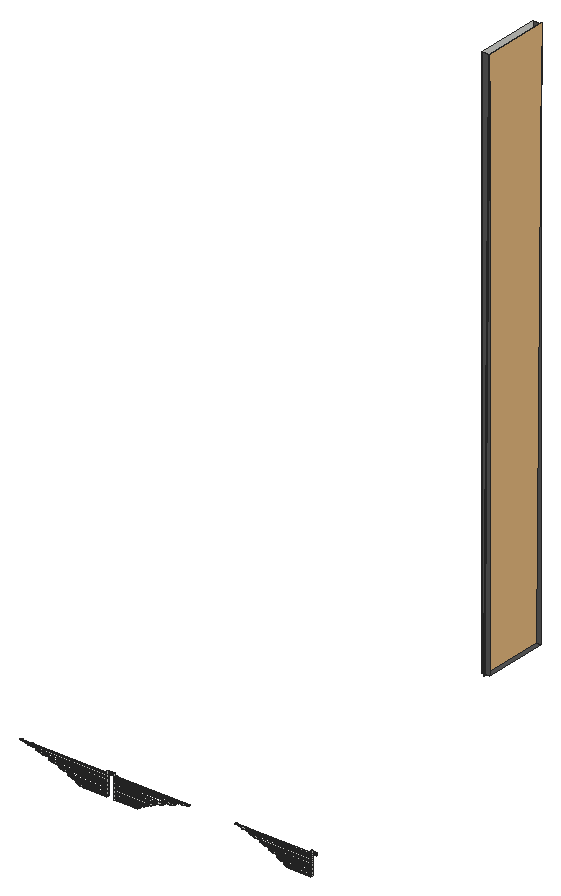
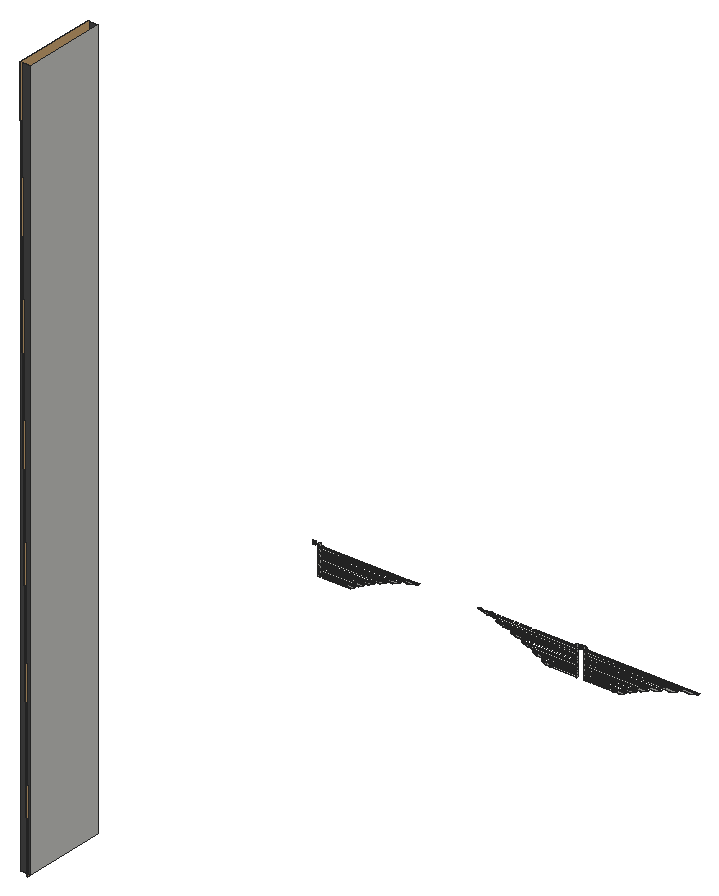
# SketchUp Ruby script. Lengths in inches.
U = 1.inch
M = Sketchup.active_model
def pt(a) = Geom::Point3d.new(a.map { |v| v * U })
def face(e, loops, mat)
  f = e.add_face(loops[0].map { |a| pt(a) })
  loops[1..].each { |l| e.add_face(l.map { |a| pt(a) }).erase! }
  f.material = f.back_material = mat if mat
  f
end
# faces: each face lists its corners as indices into pts; further lists are holes
def faces(e, pts, list, mat = nil) = list.each { |f| face(e, (f[0].is_a?(Array) ? f : [f]).map { |l| l.map { |i| pts[i] } }, mat) }
# xy, xz, yz: faces in a plane at the given z, y or x. An outline is a flat list of corners, or four numbers for a rectangle; further outlines are holes
def ring(l) = l.size == 4 ? [[l[0], l[1]], [l[2], l[1]], [l[2], l[3]], [l[0], l[3]]] : l.each_slice(2).to_a
def flat(e, list, mat, &to3) = list.each { |f| face(e, (f[0].is_a?(Array) ? f : [f]).map { |l| ring(l).map { |u, v| to3.(u, v) } }, mat) }
def xy(e, z, list, mat = nil) = flat(e, list, mat) { |x, y| [x, y, z] }
def xz(e, y, list, mat = nil) = flat(e, list, mat) { |x, z| [x, y, z] }
def yz(e, x, list, mat = nil) = flat(e, list, mat) { |y, z| [x, y, z] }
def lines(e, pts, list) = list.each { |a, b| e.add_line(pt(pts[a]), pt(pts[b])) }
# prism: a flat outline (further loops are holes) pulled along v
def prism(e, loops, v, mat = nil)
  f = face(e, loops, mat); d = Geom::Vector3d.new(v.map { |x| x * U })
  f.pushpull(f.normal.samedirection?(d) ? d.length : -d.length)
end
def box(e, o, s, mat = nil) = prism(e, [[o, [o[0] + s[0], o[1], o[2]], [o[0] + s[0], o[1] + s[1], o[2]], [o[0], o[1] + s[1], o[2]]]], [0, 0, s[2]], mat)
def at(x, y, z, deg = 0) = Geom::Transformation.translation(pt([x, y, z])) * Geom::Transformation.rotation(ORIGIN, Z_AXIS, deg.degrees)
def axes(o, x, y, z) = Geom::Transformation.new([*x, 0, *y, 0, *z, 0, *pt(o).to_a, 1])
def part(name) = M.definitions.add(name)
# library, detail: a bought-in or finely detailed component or shape, given as its bounding box
def library(name, o, s) = part(name).tap { |d| box(d.entities, o, s) }
def detail(e, o, s) = box(e.add_group.entities, o, s)
def put(e, d, t, mat = nil) = e.add_instance(d, t).tap { |i| i.material = mat if mat }
def group(e, t, mat = nil) = e.add_group.tap { |g| g.transformation = t; g.material = mat if mat }.entities
root = M.entities
M.materials.add("[Color M06]").color = [86, 86, 86]
c1 = library("Big Leaf.dwg\#1",[0,0,0],[43.17,84,0.75])
xy(root,27.6875,[[968.64,12.93,975.85,13.56],[975.85,12.93,1012.48,13.56],[1024.39,12.93,1056.27,13.56],[1056.27,12.93,1062.53,13.56],[1307.3125,12.93,1313.58,13.56],
  [1313.58,12.93,1345.46,13.56],[968.64,13.81,975.85,14.31],[975.85,13.81,1012.48,14.31],[1024.39,13.81,1056.27,14.31],[1056.27,13.81,1062.53,14.31],
  [1307.3125,13.81,1313.58,14.31],[1313.58,13.81,1345.46,14.31]])
xy(root,28.18,[[967.85,12.93,975.85,14.31],[975.85,12.93,1013.27,14.31],[1023.71,12.93,1056.27,14.31],[1056.27,12.93,1063.22,14.31],[1306.63,12.93,1313.58,14.31],
  [1313.58,12.93,1346.14,14.31]])
xy(root,30.61,[[963.14,12.93,971.13,14.31],[971.13,12.93,1013.27,14.31],[1023.71,12.93,1060.36,14.31],[1060.36,12.93,1067.32,14.31],[1302.53,12.93,1309.48,14.31],
  [1309.48,12.93,1346.14,14.31]])
xy(root,31.1,[[962.35,12.93,971.13,13.56],[971.13,12.93,1012.48,13.56],[1024.39,12.93,1060.36,13.56],[1060.36,12.93,1068,13.56],[1301.84,12.93,1309.48,13.56],
  [1309.48,12.93,1345.46,13.56],[962.35,13.81,971.13,14.31],[971.13,13.81,1012.48,14.31],[1024.39,13.81,1060.36,14.31],[1060.36,13.81,1068,14.31],
  [1301.84,13.81,1309.48,14.31],[1309.48,13.81,1345.46,14.31]])
xy(root,31.9,[[1189.6875,557.39,1202.5625,662.57]],"[Color M06]")
xy(root,33.81,[[956.23,12.93,963.95,13.56],[963.95,12.93,1012.48,13.56],[1024.39,12.93,1066.61,13.56],[1066.61,12.93,1073.33,13.56],[1296.52,12.93,1303.24,13.56],
  [1303.24,12.93,1345.46,13.56],[956.23,13.81,963.95,14.31],[963.95,13.81,1012.48,14.31],[1024.39,13.81,1066.61,14.31],[1066.61,13.81,1073.33,14.31],
  [1296.52,13.81,1303.24,14.31],[1303.24,13.81,1345.46,14.31]])
xy(root,34.3,[[955.44,12.93,963.95,14.31],[963.95,12.93,1013.27,14.31],[1023.71,12.93,1066.61,14.31],[1066.61,12.93,1074.02,14.31],[1295.83,12.93,1303.24,14.31],
  [1303.24,12.93,1346.14,14.31]])
xy(root,36.73,[[950.1,12.93,958.75,14.31],[958.75,12.93,1013.27,14.31],[1023.71,12.93,1071.14,14.31],[1071.14,12.93,1078.67,14.31],[1291.18,12.93,1298.7,14.31],
  [1298.7,12.93,1346.14,14.31]])
xy(root,37.22,[[949.3125,12.93,958.75,13.56],[958.75,12.93,1012.48,13.56],[1024.39,12.93,1071.14,13.56],[1071.14,12.93,1079.35,13.56],[1290.5,12.93,1298.7,13.56],
  [1298.7,12.93,1345.46,13.56],[949.3125,13.81,958.75,14.31],[958.75,13.81,1012.48,14.31],[1024.39,13.81,1071.14,14.31],[1071.14,13.81,1079.35,14.31],
  [1290.5,13.81,1298.7,14.31],[1298.7,13.81,1345.46,14.31]])
xy(root,39.93,[[942.21,12.93,950.6,13.56],[950.6,12.93,1012.48,13.56],[1024.39,12.93,1078.23,13.56],[1078.23,12.93,1085.53,13.56],[1284.32,12.93,1291.62,13.56],
  [1291.62,12.93,1345.46,13.56],[942.21,13.81,950.6,14.31],[950.6,13.81,1012.48,14.31],[1024.39,13.81,1078.23,14.31],[1078.23,13.81,1085.53,14.31],
  [1284.32,13.81,1291.62,14.31],[1291.62,13.81,1345.46,14.31]])
xy(root,40.42,[[941.43,12.93,950.6,14.31],[950.6,12.93,1013.27,14.31],[1023.71,12.93,1078.23,14.31],[1078.23,12.93,1086.21,14.31],[1283.64,12.93,1291.62,14.31],
  [1291.62,12.93,1346.14,14.31]])
xy(root,42.85,[[935.33,12.93,944.79,14.31],[944.79,12.93,1013.27,14.31],[1023.71,12.93,1083.28,14.31],[1083.28,12.93,1091.51,14.31],[1278.34,12.93,1286.57,14.31],
  [1286.57,12.93,1346.14,14.31]])
xy(root,43.34,[[934.55,12.93,944.79,13.56],[944.79,12.93,1012.48,13.56],[1024.39,12.93,1083.28,13.56],[1083.28,12.93,1092.19,13.56],[1277.65,12.93,1286.57,13.56],
  [1286.57,12.93,1345.46,13.56],[934.55,13.81,944.79,14.31],[944.79,13.81,1012.48,14.31],[1024.39,13.81,1083.28,14.31],[1083.28,13.81,1092.19,14.31],
  [1277.65,13.81,1286.57,14.31],[1286.57,13.81,1345.46,14.31]])
xy(root,46.05,[[926.1,12.93,935.51,13.56],[935.51,12.93,1012.48,13.56],[1024.39,12.93,1091.36,13.56],[1091.36,12.93,1099.55,13.56],[1270.3,12.93,1278.49,13.56],
  [1278.49,12.93,1345.46,13.56],[926.1,13.81,935.51,14.31],[935.51,13.81,1012.48,14.31],[1024.39,13.81,1091.36,14.31],[1091.36,13.81,1099.55,14.31],
  [1270.3,13.81,1278.49,14.31],[1278.49,13.81,1345.46,14.31]])
xy(root,46.54,[[925.31,12.93,935.51,14.31],[935.51,12.93,1013.27,14.31],[1023.71,12.93,1091.36,14.31],[1091.36,12.93,1100.23,14.31],[1269.61,12.93,1278.49,14.31],
  [1278.49,12.93,1346.14,14.31]])
xy(root,48.97,[[918.3125,12.93,928.79,14.31],[928.79,12.93,1013.27,14.31],[1023.71,12.93,1097.2,14.31],[1097.2,12.93,1106.32,14.31],[1263.53,12.93,1272.65,14.31],
  [1272.65,12.93,1346.14,14.31]])
xy(root,49.46,[[917.52,12.93,928.79,13.56],[928.79,12.93,1012.48,13.56],[1024.39,12.93,1097.2,13.56],[1097.2,12.93,1107,13.56],[1262.84,12.93,1272.65,13.56],
  [1272.65,12.93,1345.46,13.56],[917.52,13.81,928.79,14.31],[928.79,13.81,1012.48,14.31],[1024.39,13.81,1097.2,14.31],[1097.2,13.81,1107,14.31],
  [1262.84,13.81,1272.65,14.31],[1272.65,13.81,1345.46,14.31]])
xy(root,52.17,[[907.12,12.93,918.13,13.56],[918.13,12.93,1012.48,13.56],[1024.39,12.93,1106.48,13.56],[1106.48,12.93,1116.06,13.56],[1253.79,12.93,1263.37,13.56],
  [1263.37,12.93,1345.46,13.56],[907.12,13.81,918.13,14.31],[918.13,13.81,1012.48,14.31],[1024.39,13.81,1106.48,14.31],[1106.48,13.81,1116.06,14.31],
  [1253.79,13.81,1263.37,14.31],[1263.37,13.81,1345.46,14.31]])
xy(root,52.67,[[906.33,12.93,918.13,14.31],[918.13,12.93,1013.27,14.31],[1023.71,12.93,1106.48,14.31],[1106.48,12.93,1116.74,14.31],[1253.1,12.93,1263.37,14.31],
  [1263.37,12.93,1346.14,14.31]])
xy(root,55.09,[[897.86,12.93,910,14.31],[910,12.93,1013.27,14.31],[1023.71,12.93,1113.55,14.31],[1113.55,12.93,1124.11,14.31],[1245.73,12.93,1256.3,14.31],
  [1256.3,12.93,1346.14,14.31]])
xy(root,55.59,[[897.07,12.93,910,13.56],[910,12.93,1012.48,13.56],[1024.39,12.93,1113.55,13.56],[1113.55,12.93,1124.8,13.56],[1245.05,12.93,1256.3,13.56],
  [1256.3,12.93,1345.46,13.56],[897.07,13.81,910,14.31],[910,13.81,1012.48,14.31],[1024.39,13.81,1113.55,14.31],[1113.55,13.81,1124.8,14.31],
  [1245.05,13.81,1256.3,14.31],[1256.3,13.81,1345.46,14.31]])
xy(root,58.29,[[884.76,12.93,896.8,13.56],[896.8,12.93,1012.48,13.56],[1024.39,12.93,1125.03,13.56],[1125.03,12.93,1135.51,13.56],[1234.34,12.93,1244.82,13.56],
  [1244.82,12.93,1345.46,13.56],[884.76,13.81,896.8,14.31],[896.8,13.81,1012.48,14.31],[1024.39,13.81,1125.03,14.31],[1125.03,13.81,1135.51,14.31],
  [1234.34,13.81,1244.82,14.31],[1244.82,13.81,1345.46,14.31]])
xy(root,58.79,[[896.8,12.93,1013.27,14.31],[1023.71,12.93,1125.03,14.31],[1244.82,12.93,1346.14,14.31]])
xy(root,61.21,[[871.53,12.93,887.21,14.31],[887.21,12.93,1013.27,14.31],[1023.71,12.93,1133.375,14.31],[1133.375,12.93,1147.02,14.31],[1222.82,12.93,1236.47,14.31],
  [1236.47,12.93,1346.14,14.31]])
xy(root,61.46,[[1014.6875,13.24,1018.58,14.43],[1019.16,13.24,1023.63,14.43],[1351.27,13.24,1355.16,14.43]])
xy(root,61.71,[[870.74,12.93,887.21,13.56],[887.21,12.93,1012.48,13.56],[1024.39,12.93,1133.375,13.56],[1133.375,12.93,1147.71,13.56],[1222.14,12.93,1236.47,13.56],
  [1236.47,12.93,1345.46,13.56],[870.74,13.81,887.21,14.31],[887.21,13.81,1012.48,14.31],[1024.39,13.81,1133.375,14.31],[1133.375,13.81,1147.71,14.31],
  [1222.14,13.81,1236.47,14.31],[1236.47,13.81,1345.46,14.31]])
xy(root,62.75,[[1014.6875,13.24,1018.58,14.43],[1019.16,13.24,1023.63,14.43],[1351.27,13.24,1355.16,14.43]])
xy(root,63.67,[[1014.6875,13.24,1018.58,14.43],[1019.16,13.24,1023.63,14.43],[1351.27,13.24,1355.16,14.43]])
xz(root,12.93,[[967.85,28.18,963.14,30.61,971.13,30.61,975.85,28.18],[1056.27,28.18,1063.22,28.18,1067.32,30.61,1060.36,30.61],[1306.63,28.18,1302.53,30.61,1309.48,30.61,1313.58,28.18],[955.44,34.3,950.1,36.73,958.75,36.73,962.94,34.82,963.95,34.3],[1066.61,34.3,1074.02,34.3,1078.67,36.73,1071.14,36.73,1067.49,34.82],
  [1295.83,34.3,1291.18,36.73,1298.7,36.73,1302.36,34.82,1303.24,34.3],[941.43,40.42,935.33,42.85,944.79,42.85,948.59,41.34,950.6,40.42],[1078.23,40.42,1086.21,40.42,1091.51,42.85,1083.28,42.85,1079.97,41.34],[1283.64,40.42,1278.34,42.85,1286.57,42.85,1289.87,41.34,1291.62,40.42],[925.31,46.54,918.3125,48.97,928.79,48.97,933.64,47.29,935.51,46.54],
  [1091.36,46.54,1100.23,46.54,1106.32,48.97,1097.2,48.97,1092.98,47.29],[1269.61,46.54,1263.53,48.97,1272.65,48.97,1276.86,47.29,1278.49,46.54],[906.33,52.67,900.11,54.52,897.86,55.09,910,55.09,918.13,52.67],[1106.48,52.67,1116.74,52.67,1122.15,54.52,1124.11,55.09,1113.55,55.09],[1253.1,52.67,1247.69,54.52,1245.73,55.09,1256.3,55.09,1263.37,52.67],
  [883.97,58.6,883.1,58.79,871.53,61.21,887.21,61.21,896.8,58.79,883.97,58.79],[1136.19,58.6,1136.96,58.79,1147.02,61.21,1133.375,61.21,1125.03,58.79,1136.19,58.79],[1233.65,58.6,1232.89,58.79,1222.82,61.21,1236.47,61.21,1244.82,58.79,1233.65,58.79]])
xz(root,13.24,[[1014.6875,61.46,1018.58,62.75],[1019.16,61.46,1023.63,62.75],[1351.27,61.46,1355.16,62.75],[1014.6875,63.67,1018.58,64.96],[1019.16,63.67,1023.63,64.96],
  [1351.27,63.67,1355.16,64.96]])
xz(root,14.31,[[967.85,28.18,975.85,28.18,971.13,30.61,963.14,30.61],[1056.27,28.18,1060.36,30.61,1067.32,30.61,1063.22,28.18],[1306.63,28.18,1313.58,28.18,1309.48,30.61,1302.53,30.61],[955.44,34.3,963.95,34.3,962.94,34.82,958.75,36.73,950.1,36.73],[1066.61,34.3,1067.49,34.82,1071.14,36.73,1078.67,36.73,1074.02,34.3],
  [1295.83,34.3,1303.24,34.3,1302.36,34.82,1298.7,36.73,1291.18,36.73],[941.43,40.42,950.6,40.42,948.59,41.34,944.79,42.85,935.33,42.85],[1078.23,40.42,1079.97,41.34,1083.28,42.85,1091.51,42.85,1086.21,40.42],[1283.64,40.42,1291.62,40.42,1289.87,41.34,1286.57,42.85,1278.34,42.85],[925.31,46.54,935.51,46.54,933.64,47.29,928.79,48.97,918.3125,48.97],
  [1091.36,46.54,1092.98,47.29,1097.2,48.97,1106.32,48.97,1100.23,46.54],[1269.61,46.54,1278.49,46.54,1276.86,47.29,1272.65,48.97,1263.53,48.97],[906.33,52.67,918.13,52.67,910,55.09,897.86,55.09,900.11,54.52],[1106.48,52.67,1113.55,55.09,1124.11,55.09,1122.15,54.52,1116.74,52.67],[1253.1,52.67,1263.37,52.67,1256.3,55.09,1245.73,55.09,1247.69,54.52],
  [883.97,58.6,883.97,58.79,896.8,58.79,887.21,61.21,871.53,61.21,883.1,58.79],[1136.19,58.6,1136.19,58.79,1125.03,58.79,1133.375,61.21,1147.02,61.21,1136.96,58.79],[1233.65,58.6,1233.65,58.79,1244.82,58.79,1236.47,61.21,1222.82,61.21,1232.89,58.79]])
xz(root,14.43,[[1014.6875,61.46,1018.58,62.75],[1019.16,61.46,1023.63,62.75],[1351.27,61.46,1355.16,62.75],[1014.6875,63.67,1018.58,64.96],[1019.16,63.67,1023.63,64.96],
  [1351.27,63.67,1355.16,64.96]])
xz(root,557.39,[[1189.6875,31.9,1202.5625,941.41]],"[Color M06]")
xz(root,662.57,[[1189.6875,31.9,1202.5625,941.41]],"[Color M06]")
yz(root,1012.48,[[12.93,31.1,13.56,33.81],[13.81,31.1,14.31,33.81],[12.93,37.22,13.56,39.93],[13.81,37.22,14.31,39.93],[12.93,43.34,13.56,46.05],
  [13.81,43.34,14.31,46.05],[12.93,49.46,13.56,52.17],[13.81,49.46,14.31,52.17],[12.93,55.59,13.56,58.29],[13.81,55.59,14.31,58.29],
  [12.93,61.71,13.56,64.41],[13.81,61.71,14.31,64.41]])
yz(root,1013.27,[[12.93,30.61,14.31,34.3],[14.31,30.61,15.56,34.3],[12.93,36.73,14.31,40.42],[14.31,36.73,15.56,40.42],[12.93,42.85,14.31,46.54],
  [14.31,42.85,15.56,46.54],[12.93,48.97,14.31,52.67],[14.31,48.97,15.56,52.67],[12.93,55.09,14.31,58.79],[14.31,55.09,15.56,58.79],
  [12.93,61.21,14.31,64.91],[14.31,61.21,15.56,64.91]])
yz(root,1014.39,[[14.12,28.18,15.56,30.61],[14.12,30.61,15.56,34.3],[14.12,34.3,15.56,36.73],[14.12,36.73,15.56,40.42],[14.12,40.42,15.56,42.85],
  [14.12,42.85,15.56,46.54],[14.12,46.54,15.56,48.97],[14.12,48.97,15.56,52.67],[14.12,52.67,15.56,55.09],[14.12,55.09,15.56,58.79],
  [14.12,58.79,15.56,61.21],[14.12,61.21,15.56,64.91]])
yz(root,1014.6875,[[13.24,61.46,14.43,62.75],[13.24,63.67,14.43,64.96]])
yz(root,1022.73,[[14.12,28.18,15.56,30.61],[14.12,30.61,15.56,34.3],[14.12,34.3,15.56,36.73],[14.12,36.73,15.56,40.42],[14.12,40.42,15.56,42.85],
  [14.12,42.85,15.56,46.54],[14.12,46.54,15.56,48.97],[14.12,48.97,15.56,52.67],[14.12,52.67,15.56,55.09],[14.12,55.09,15.56,58.79],
  [14.12,58.79,15.56,61.21],[14.12,61.21,15.56,64.91]])
yz(root,1023.63,[[13.24,61.46,14.43,62.75],[13.24,63.67,14.43,64.96]])
yz(root,1023.71,[[12.93,30.61,14.31,34.3],[14.31,30.61,15.56,34.3],[12.93,36.73,14.31,40.42],[14.31,36.73,15.56,40.42],[12.93,42.85,14.31,46.54],
  [14.31,42.85,15.56,46.54],[12.93,48.97,14.31,52.67],[14.31,48.97,15.56,52.67],[12.93,55.09,14.31,58.79],[14.31,55.09,15.56,58.79],
  [12.93,61.21,14.31,64.91],[14.31,61.21,15.56,64.91]])
yz(root,1024.39,[[12.93,31.1,13.56,33.81],[13.81,31.1,14.31,33.81],[12.93,37.22,13.56,39.93],[13.81,37.22,14.31,39.93],[12.93,43.34,13.56,46.05],
  [13.81,43.34,14.31,46.05],[12.93,49.46,13.56,52.17],[13.81,49.46,14.31,52.17],[12.93,55.59,13.56,58.29],[13.81,55.59,14.31,58.29],
  [12.93,61.71,13.56,64.41],[13.81,61.71,14.31,64.41]])
yz(root,1189.6875,[[557.39,31.9,662.57,941.41]])
yz(root,1345.46,[[12.93,31.1,13.56,33.81],[13.81,31.1,14.31,33.81],[12.93,37.22,13.56,39.93],[13.81,37.22,14.31,39.93],[12.93,43.34,13.56,46.05],
  [13.81,43.34,14.31,46.05],[12.93,49.46,13.56,52.17],[13.81,49.46,14.31,52.17],[12.93,55.59,13.56,58.29],[13.81,55.59,14.31,58.29],
  [12.93,61.71,13.56,64.41],[13.81,61.71,14.31,64.41]])
yz(root,1346.14,[[12.93,30.61,14.31,34.3],[14.31,30.61,15.56,34.3],[12.93,36.73,14.31,40.42],[14.31,36.73,15.56,40.42],[12.93,42.85,14.31,46.54],
  [14.31,42.85,15.56,46.54],[12.93,48.97,14.31,52.67],[14.31,48.97,15.56,52.67],[12.93,55.09,14.31,58.79],[14.31,55.09,15.56,58.79],
  [12.93,61.21,14.31,64.91],[14.31,61.21,15.56,64.91]])
yz(root,1347.11,[[14.12,28.18,15.56,30.61],[14.12,30.61,15.56,34.3],[14.12,34.3,15.56,36.73],[14.12,36.73,15.56,40.42],[14.12,40.42,15.56,42.85],
  [14.12,42.85,15.56,46.54],[14.12,46.54,15.56,48.97],[14.12,48.97,15.56,52.67],[14.12,52.67,15.56,55.09],[14.12,55.09,15.56,58.79],
  [14.12,58.79,15.56,61.21],[14.12,61.21,15.56,64.91]])
yz(root,1355.16,[[13.24,61.46,14.43,62.75],[13.24,63.67,14.43,64.96]])
p = [[967.85,14.31,28.18],[963.14,14.31,30.61],[963.14,12.93,30.61],[967.85,12.93,28.18],[971.13,14.31,30.61],[975.85,14.31,28.18],
  [975.85,12.93,28.18],[971.13,12.93,30.61],[1060.36,14.31,30.61],[1056.27,14.31,28.18],[1056.27,12.93,28.18],[1060.36,12.93,30.61],
  [1063.22,14.31,28.18],[1067.32,14.31,30.61],[1067.32,12.93,30.61],[1063.22,12.93,28.18],[1306.63,14.31,28.18],[1302.53,14.31,30.61],
  [1302.53,12.93,30.61],[1306.63,12.93,28.18],[1309.48,14.31,30.61],[1313.58,14.31,28.18],[1313.58,12.93,28.18],[1309.48,12.93,30.61],
  [955.44,14.31,34.3],[950.1,14.31,36.73],[950.1,12.93,36.73],[955.44,12.93,34.3],[962.94,14.31,34.82],[963.95,14.31,34.3],
  [963.95,12.93,34.3],[962.94,12.93,34.82],[1067.49,14.31,34.82],[1066.61,14.31,34.3],[1066.61,12.93,34.3],[1067.49,12.93,34.82],
  [1074.02,14.31,34.3],[1078.67,14.31,36.73],[1078.67,12.93,36.73],[1074.02,12.93,34.3],[1295.83,14.31,34.3],[1291.18,14.31,36.73],
  [1291.18,12.93,36.73],[1295.83,12.93,34.3],[1302.36,14.31,34.82],[1303.24,14.31,34.3],[1303.24,12.93,34.3],[1302.36,12.93,34.82],
  [958.75,14.31,36.73],[958.75,12.93,36.73],[1071.14,14.31,36.73],[1071.14,12.93,36.73],[1298.7,14.31,36.73],[1298.7,12.93,36.73],
  [941.43,14.31,40.42],[935.33,14.31,42.85],[935.33,12.93,42.85],[941.43,12.93,40.42],[948.59,14.31,41.34],[950.6,14.31,40.42],
  [950.6,12.93,40.42],[948.59,12.93,41.34],[1079.97,14.31,41.34],[1078.23,14.31,40.42],[1078.23,12.93,40.42],[1079.97,12.93,41.34],
  [1086.21,14.31,40.42],[1091.51,14.31,42.85],[1091.51,12.93,42.85],[1086.21,12.93,40.42],[1283.64,14.31,40.42],[1278.34,14.31,42.85],
  [1278.34,12.93,42.85],[1283.64,12.93,40.42],[1289.87,14.31,41.34],[1291.62,14.31,40.42],[1291.62,12.93,40.42],[1289.87,12.93,41.34],
  [944.79,14.31,42.85],[944.79,12.93,42.85],[1083.28,14.31,42.85],[1083.28,12.93,42.85],[1286.57,14.31,42.85],[1286.57,12.93,42.85],
  [925.31,14.31,46.54],[918.3125,14.31,48.97],[918.3125,12.93,48.97],[925.31,12.93,46.54],[933.64,14.31,47.29],[935.51,14.31,46.54],
  [935.51,12.93,46.54],[933.64,12.93,47.29],[1092.98,14.31,47.29],[1091.36,14.31,46.54],[1091.36,12.93,46.54],[1092.98,12.93,47.29],
  [1100.23,14.31,46.54],[1106.32,14.31,48.97],[1106.32,12.93,48.97],[1100.23,12.93,46.54],[1269.61,14.31,46.54],[1263.53,14.31,48.97],
  [1263.53,12.93,48.97],[1269.61,12.93,46.54],[1276.86,14.31,47.29],[1278.49,14.31,46.54],[1278.49,12.93,46.54],[1276.86,12.93,47.29],
  [928.79,14.31,48.97],[928.79,12.93,48.97],[1097.2,14.31,48.97],[1097.2,12.93,48.97],[1272.65,14.31,48.97],[1272.65,12.93,48.97],
  [906.33,14.31,52.67],[900.11,14.31,54.52],[900.11,12.93,54.52],[906.33,12.93,52.67],[910,14.31,55.09],[918.13,14.31,52.67],
  [918.13,12.93,52.67],[910,12.93,55.09],[1113.55,14.31,55.09],[1106.48,14.31,52.67],[1106.48,12.93,52.67],[1113.55,12.93,55.09],
  [1116.74,14.31,52.67],[1122.15,14.31,54.52],[1122.15,12.93,54.52],[1116.74,12.93,52.67],[1253.1,14.31,52.67],[1247.69,14.31,54.52],
  [1247.69,12.93,54.52],[1253.1,12.93,52.67],[1256.3,14.31,55.09],[1263.37,14.31,52.67],[1263.37,12.93,52.67],[1256.3,12.93,55.09],
  [897.86,14.31,55.09],[897.86,12.93,55.09],[1124.11,14.31,55.09],[1124.11,12.93,55.09],[1245.73,14.31,55.09],[1245.73,12.93,55.09],
  [883.97,14.31,58.6],[883.1,14.31,58.79],[871.53,14.31,61.21],[871.53,12.93,61.21],[883.1,12.93,58.79],[883.97,12.93,58.6],
  [1136.19,14.31,58.6],[1136.96,14.31,58.79],[1147.02,14.31,61.21],[1147.02,12.93,61.21],[1136.96,12.93,58.79],[1136.19,12.93,58.6],
  [1233.65,14.31,58.6],[1232.89,14.31,58.79],[1222.82,14.31,61.21],[1222.82,12.93,61.21],[1232.89,12.93,58.79],[1233.65,12.93,58.6],
  [887.21,14.31,61.21],[896.8,14.31,58.79],[896.8,12.93,58.79],[887.21,12.93,61.21],[1133.375,14.31,61.21],[1125.03,14.31,58.79],
  [1125.03,12.93,58.79],[1133.375,12.93,61.21],[1236.47,14.31,61.21],[1244.82,14.31,58.79],[1244.82,12.93,58.79],[1236.47,12.93,61.21]]
faces(root,p,[[0,1,2,3],[4,5,6,7],[8,9,10,11],[12,13,14,15],[16,17,18,19],[20,21,22,23],[24,25,26,27],[28,29,30,31],
  [32,33,34,35],[36,37,38,39],[40,41,42,43],[44,45,46,47],[48,28,31,49],[50,32,35,51],[52,44,47,53],[54,55,56,57],
  [58,59,60,61],[62,63,64,65],[66,67,68,69],[70,71,72,73],[74,75,76,77],[78,58,61,79],[80,62,65,81],[82,74,77,83],
  [84,85,86,87],[88,89,90,91],[92,93,94,95],[96,97,98,99],[100,101,102,103],[104,105,106,107],[108,88,91,109],[110,92,95,111],
  [112,104,107,113],[114,115,116,117],[118,119,120,121],[122,123,124,125],[126,127,128,129],[130,131,132,133],[134,135,136,137],[115,138,139,116],
  [127,140,141,128],[131,142,143,132],[144,145,146,147,148,149],[150,151,152,153,154,155],[156,157,158,159,160,161],[162,163,164,165],[166,167,168,169],[170,171,172,173]])
put(root,c1,axes([1201.8125,663.6,941.42],[0,-2.46,0],[-0.10001,0,-10.85954],[0.99996,0,-0.00921]))
